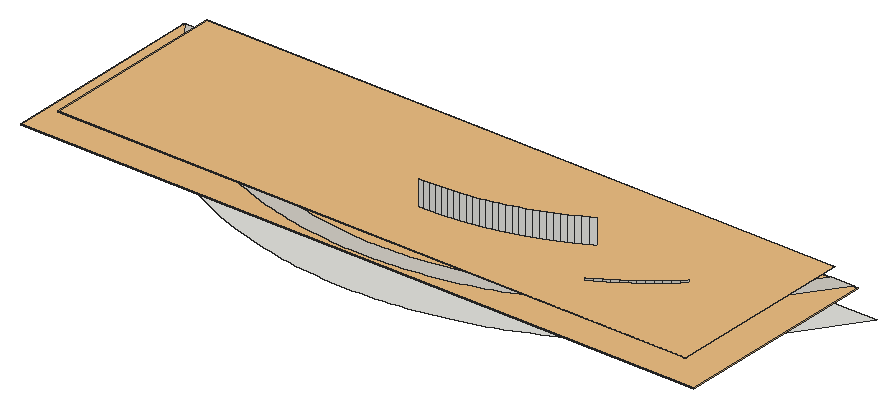
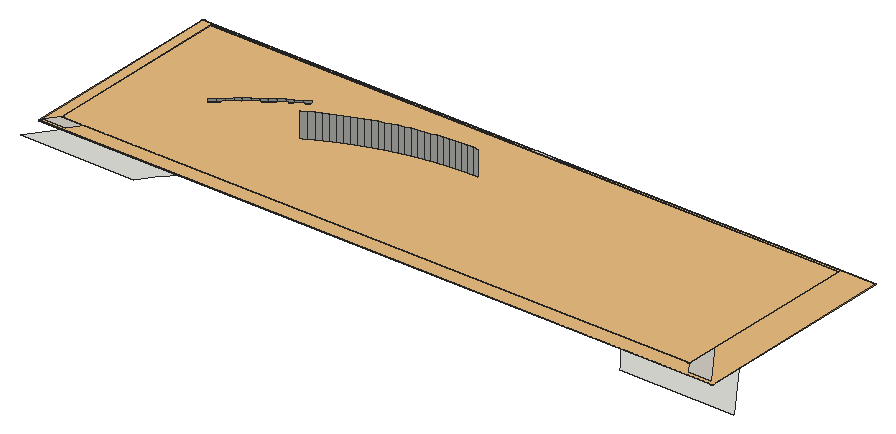
# SketchUp Ruby script. Lengths in inches.
U = 1.inch
M = Sketchup.active_model
def pt(a) = Geom::Point3d.new(a.map { |v| v * U })
def face(e, loops, mat)
  f = e.add_face(loops[0].map { |a| pt(a) })
  loops[1..].each { |l| e.add_face(l.map { |a| pt(a) }).erase! }
  f.material = f.back_material = mat if mat
  f
end
# faces: each face lists its corners as indices into pts; further lists are holes
def faces(e, pts, list, mat = nil) = list.each { |f| face(e, (f[0].is_a?(Array) ? f : [f]).map { |l| l.map { |i| pts[i] } }, mat) }
# xy, xz, yz: faces in a plane at the given z, y or x. An outline is a flat list of corners, or four numbers for a rectangle; further outlines are holes
def ring(l) = l.size == 4 ? [[l[0], l[1]], [l[2], l[1]], [l[2], l[3]], [l[0], l[3]]] : l.each_slice(2).to_a
def flat(e, list, mat, &to3) = list.each { |f| face(e, (f[0].is_a?(Array) ? f : [f]).map { |l| ring(l).map { |u, v| to3.(u, v) } }, mat) }
def xy(e, z, list, mat = nil) = flat(e, list, mat) { |x, y| [x, y, z] }
def xz(e, y, list, mat = nil) = flat(e, list, mat) { |x, z| [x, y, z] }
def yz(e, x, list, mat = nil) = flat(e, list, mat) { |y, z| [x, y, z] }
def lines(e, pts, list) = list.each { |a, b| e.add_line(pt(pts[a]), pt(pts[b])) }
# prism: a flat outline (further loops are holes) pulled along v
def prism(e, loops, v, mat = nil)
  f = face(e, loops, mat); d = Geom::Vector3d.new(v.map { |x| x * U })
  f.pushpull(f.normal.samedirection?(d) ? d.length : -d.length)
end
def box(e, o, s, mat = nil) = prism(e, [[o, [o[0] + s[0], o[1], o[2]], [o[0] + s[0], o[1] + s[1], o[2]], [o[0], o[1] + s[1], o[2]]]], [0, 0, s[2]], mat)
def at(x, y, z, deg = 0) = Geom::Transformation.translation(pt([x, y, z])) * Geom::Transformation.rotation(ORIGIN, Z_AXIS, deg.degrees)
def axes(o, x, y, z) = Geom::Transformation.new([*x, 0, *y, 0, *z, 0, *pt(o).to_a, 1])
def part(name) = M.definitions.add(name)
# library, detail: a bought-in or finely detailed component or shape, given as its bounding box
def library(name, o, s) = part(name).tap { |d| box(d.entities, o, s) }
def detail(e, o, s) = box(e.add_group.entities, o, s)
def put(e, d, t, mat = nil) = e.add_instance(d, t).tap { |i| i.material = mat if mat }
def group(e, t, mat = nil) = e.add_group.tap { |g| g.transformation = t; g.material = mat if mat }.entities
root = M.entities
M.materials.add("Arta-Ceramic-Moonstone-White-24x24-4K").color = [209, 205, 196]
c1 = library("Mesh Light\#8",[-0.5,-0.5,-0.1],[1,1,0.2])
c2 = library("Mesh Light\#7",[-0.5,-0.5,-0.1],[1,1,0.2])
xy(root,0,[[1024.28,79.26,1020.34,79.3,1016.39,79.42,1012.45,79.6,1008.51,79.87,1004.58,80.21,1000.66,80.625,996.74,81.12,992.84,81.68,988.94,82.32,985.0625,83.04,981.2,83.83,977.35,84.69,973.51,85.63,969.7,86.64,965.91,87.72,962.13,88.88,958.38,90.11,954.66,91.41,950.96,92.78,947.29,94.22,943.64,95.73,940.03,97.32,936.44,98.97,932.89,100.6875,929.37,102.47,925.89,104.33,922.44,106.25,919.03,108.24,915.66,110.29,912.33,112.4,909.04,114.58,905.8,116.82,902.59,119.13,899.44,121.49,896.32,123.92,893.26,126.4,890.24,128.95,887.27,131.55,884.36,134.2,881.49,136.92,878.68,139.68,875.92,142.5,873.21,145.375,870.5625,148.3,867.97,151.27,865.43,154.3,862.96,157.37,860.54,160.49,858.18,163.65,835.84,194.875,895.84,194.875,897.59,192.43,899.39,190.01,901.24,187.64,903.125,185.29,905.06,182.99,907.04,180.72,909.06,178.49,911.12,176.3,913.23,174.15,915.37,172.04,917.56,169.97,919.78,167.94,922.05,165.96,924.35,164.02,926.69,162.12,929.06,160.27,931.47,158.47,933.91,156.71,936.39,155,938.9,153.34,941.4375,151.72,944.01,150.16,946.61,148.64,949.24,147.18,951.89,145.76,954.58,144.4,957.28,143.09,960.02,141.83,962.78,140.625,965.56,139.47,968.36,138.37,971.18,137.32,974.02,136.33,976.88,135.4,979.76,134.51,982.65,133.6875,985.56,132.92,988.48,132.2,991.42,131.54,994.37,130.94,997.33,130.4,1000.3,129.91,1003.28,129.48,1006.26,129.1,1009.26,128.78,1012.25,128.52,1015.26,128.32,1018.26,128.18,1021.27,128.09,1024.28,128.0625,1027.29,128.09,1030.3,128.18,1033.3,128.32,1036.31,128.52,1039.31,128.78,1042.3,129.1,1045.28,129.48,1048.26,129.91,1051.23,130.4,1054.19,130.94,1057.14,131.54,1060.08,132.2,1063,132.92,1065.91,133.6875,1068.8,134.51,1071.68,135.4,1074.54,136.33,1077.38,137.32,1080.21,138.37,1083.01,139.47,1085.79,140.625,1088.54,141.83,1091.28,143.09,1093.99,144.4,1096.67,145.76,1099.33,147.18,1101.95,148.64,1104.55,150.16,1107.125,151.72,1109.67,153.34,1112.17,155,1114.65,156.71,1117.09,158.47,1119.5,160.27,1121.875,162.12,1124.21,164.02,1126.52,165.96,1128.78,167.94,1131,169.97,1133.19,172.04,1135.34,174.15,1137.44,176.3,1139.5,178.49,1141.52,180.72,1143.5,182.99,1145.4375,185.29,1147.33,187.64,1149.17,190.01,1150.97,192.43,1152.72,194.875,1212.72,194.875,1190.38,163.65,1188.02,160.49,1185.6,157.37,1183.13,154.3,1180.59,151.27,1178,148.3,1175.35,145.375,1172.65,142.5,1169.89,139.68,1167.07,136.92,1164.21,134.2,1161.29,131.55,1158.32,128.95,1155.3,126.4,1152.24,123.92,1149.125,121.49,1145.97,119.13,1142.76,116.82,1139.52,114.58,1136.23,112.4,1132.9,110.29,1129.53,108.24,1126.12,106.25,1122.67,104.33,1119.1875,102.47,1115.67,100.6875,1112.12,98.97,1108.54,97.32,1104.92,95.73,1101.28,94.22,1097.6,92.78,1093.9,91.41,1090.18,90.11,1086.43,88.88,1082.66,87.72,1078.86,86.64,1075.05,85.63,1071.21,84.69,1067.36,83.83,1063.5,83.04,1059.62,82.32,1055.72,81.68,1051.82,81.12,1047.9,80.625,1043.98,80.21,1040.05,79.87,1036.11,79.6,1032.17,79.42,1028.23,79.3]])
xy(root,12,[[1024.28,89.02,1028.04,89.06,1031.8,89.17,1035.55,89.35,1039.3,89.6,1043.05,89.92,1046.78,90.32,1050.51,90.79,1054.23,91.33,1057.94,91.9375,1061.64,92.62,1065.32,93.37,1068.99,94.19,1072.64,95.09,1076.27,96.05,1079.89,97.08,1083.48,98.18,1087.05,99.35,1090.6,100.59,1094.125,101.9,1097.62,103.27,1101.09,104.71,1104.54,106.22,1107.95,107.79,1111.33,109.43,1114.68,111.13,1118,112.9,1121.29,114.73,1124.53,116.62,1127.74,118.57,1130.92,120.59,1134.05,122.67,1137.14,124.8,1140.19,127,1143.2,129.25,1146.17,131.56,1149.09,133.93,1151.96,136.35,1154.79,138.83,1157.57,141.36,1160.3,143.94,1162.98,146.58,1165.6,149.26,1168.18,152,1170.7,154.78,1173.17,157.62,1175.59,160.5,1177.95,163.42,1180.25,166.39,1182.5,169.41,1200.72,194.875,1188.72,194.875,1174.61,175.16,1172.48,172.3,1170.29,169.48,1168.05,166.7,1165.76,163.96,1163.41,161.27,1161.01,158.62,1158.5625,156.02,1156.07,153.47,1153.52,150.96,1150.93,148.51,1148.29,146.1,1145.6,143.75,1142.87,141.45,1140.09,139.2,1137.28,137.01,1134.42,134.86,1131.52,132.78,1128.58,130.75,1125.6,128.78,1122.59,126.86,1119.54,125,1116.45,123.21,1113.33,121.47,1110.18,119.79,1107,118.17,1103.78,116.62,1100.54,115.12,1097.27,113.69,1093.97,112.32,1090.64,111.02,1087.3,109.77,1083.92,108.6,1080.53,107.49,1077.12,106.4375,1073.68,105.46,1070.23,104.54,1066.76,103.7,1063.28,102.91,1059.78,102.2,1056.26,101.55,1052.74,100.97,1049.21,100.46,1045.66,100.02,1042.11,99.64,1038.55,99.33,1034.99,99.09,1031.42,98.92,1027.85,98.82,1024.28,98.78,1020.71,98.82,1017.14,98.92,1013.57,99.09,1010.01,99.33,1006.45,99.64,1002.9,100.02,999.36,100.46,995.82,100.97,992.3,101.55,988.79,102.2,985.29,102.91,981.8,103.7,978.33,104.54,974.88,105.46,971.45,106.4375,968.03,107.49,964.64,108.6,961.27,109.77,957.92,111.02,954.59,112.32,951.29,113.69,948.02,115.12,944.78,116.62,941.56,118.17,938.38,119.79,935.23,121.47,932.11,123.21,929.02,125,925.97,126.86,922.96,128.78,919.98,130.75,917.04,132.78,914.14,134.86,911.28,137.01,908.47,139.2,905.69,141.45,902.96,143.75,900.28,146.1,897.64,148.51,895.04,150.96,892.5,153.47,890,156.02,887.55,158.62,885.15,161.27,882.81,163.96,880.51,166.7,878.27,169.48,876.08,172.3,873.95,175.16,859.84,194.875,847.84,194.875,866.06,169.41,868.31,166.39,870.61,163.42,872.97,160.5,875.39,157.62,877.86,154.78,880.38,152,882.96,149.26,885.59,146.58,888.27,143.94,891,141.36,893.77,138.83,896.6,136.35,899.48,133.93,902.4,131.56,905.36,129.25,908.37,127,911.42,124.8,914.51,122.67,917.65,120.59,920.82,118.57,924.03,116.62,927.28,114.73,930.56,112.9,933.875,111.13,937.23,109.43,940.61,107.79,944.02,106.22,947.47,104.71,950.9375,103.27,954.4375,101.9,957.96,100.59,961.51,99.35,965.08,98.18,968.68,97.08,972.29,96.05,975.92,95.09,979.57,94.19,983.24,93.37,986.92,92.62,990.62,91.9375,994.33,91.33,998.05,90.79,1001.78,90.32,1005.52,89.92,1009.26,89.6,1013.01,89.35,1016.77,89.17,1020.52,89.06]],"Arta-Ceramic-Moonstone-White-24x24-4K")
p = [[1152.24,123.92,5],[1152.24,123.92,0],[1155.3,126.4,0],[1155.3,126.4,5],[1158.32,128.95,0],[1158.32,128.95,5],
  [1024.28,128.0625,0],[1024.28,128.0625,30],[1027.29,128.09,30],[1027.29,128.09,0],[1030.3,128.18,30],[1030.3,128.18,0],
  [1033.3,128.32,30],[1033.3,128.32,0],[1036.31,128.52,30],[1036.31,128.52,0],[1039.31,128.78,30],[1039.31,128.78,0],
  [1042.3,129.1,30],[1042.3,129.1,0],[1161.29,131.55,0],[1161.29,131.55,5],[1045.28,129.48,30],[1045.28,129.48,0],
  [1048.26,129.91,30],[1048.26,129.91,0],[1051.23,130.4,30],[1051.23,130.4,0],[1054.19,130.94,30],[1054.19,130.94,0],
  [1057.14,131.54,30],[1057.14,131.54,0],[1060.08,132.2,30],[1060.08,132.2,0],[1164.21,134.2,0],[1164.21,134.2,5],
  [1063,132.92,30],[1063,132.92,0],[1065.91,133.6875,30],[1065.91,133.6875,0],[1068.8,134.51,30],[1068.8,134.51,0],
  [1167.07,136.92,0],[1167.07,136.92,5],[1071.68,135.4,30],[1071.68,135.4,0],[1074.54,136.33,30],[1074.54,136.33,0],
  [1077.38,137.32,30],[1077.38,137.32,0],[1169.89,139.68,0],[1169.89,139.68,5],[1080.21,138.37,30],[1080.21,138.37,0],
  [1083.01,139.47,30],[1083.01,139.47,0],[1085.79,140.625,30],[1085.79,140.625,0],[1172.65,142.5,0],[1172.65,142.5,5],
  [1088.54,141.83,30],[1088.54,141.83,0],[1091.28,143.09,30],[1091.28,143.09,0],[1175.35,145.375,0],[1175.35,145.375,5],
  [1093.99,144.4,30],[1093.99,144.4,0],[1096.67,145.76,30],[1096.67,145.76,0],[1178,148.3,0],[1178,148.3,5],
  [1099.33,147.18,30],[1099.33,147.18,0],[1101.95,148.64,30],[1101.95,148.64,0],[1152.74,123.28,6],[1152.74,123.28,5],
  [1155.82,125.78,5],[1155.82,125.78,6],[1158.85,128.33,5],[1158.85,128.33,6],[1161.83,130.94,5],[1161.83,130.94,6],
  [1164.76,133.61,5],[1164.76,133.61,6],[1167.64,136.33,5],[1167.64,136.33,6],[1170.46,139.11,5],[1170.46,139.11,6],
  [1173.23,141.94,5],[1173.23,141.94,6],[1175.95,144.82,5],[1175.95,144.82,6],[1178.61,147.76,5],[1178.61,147.76,6],
  [1134.05,122.67,11],[1134.05,122.67,6],[1137.14,124.8,6],[1137.14,124.8,11],[1140.19,127,6],[1140.19,127,11],
  [1143.2,129.25,6],[1143.2,129.25,11],[1146.17,131.56,6],[1146.17,131.56,11],[1149.09,133.93,6],[1149.09,133.93,11],
  [1151.96,136.35,6],[1151.96,136.35,11],[1154.79,138.83,6],[1154.79,138.83,11],[1157.57,141.36,6],[1157.57,141.36,11],
  [1160.3,143.94,6],[1160.3,143.94,11],[1162.98,146.58,6],[1162.98,146.58,11],[1165.6,149.26,6],[1165.6,149.26,11],
  [1134.5,121.99,12],[1134.5,121.99,11],[1137.61,124.14,11],[1137.61,124.14,12],[1140.67,126.34,11],[1140.67,126.34,12],
  [1143.7,128.6,11],[1143.7,128.6,12],[1146.67,130.92,11],[1146.67,130.92,12],[1149.6,133.3,11],[1149.6,133.3,12],
  [1152.49,135.73,11],[1152.49,135.73,12],[1155.33,138.22,11],[1155.33,138.22,12],[1158.12,140.76,11],[1158.12,140.76,12],
  [1160.86,143.35,11],[1160.86,143.35,12],[1163.55,146,11],[1163.55,146,12],[1166.19,148.7,11],[1166.19,148.7,12],
  [1116.45,123.21,17],[1116.45,123.21,12],[1119.54,125,12],[1119.54,125,17],[1122.59,126.86,12],[1122.59,126.86,17],
  [1125.6,128.78,12],[1125.6,128.78,17],[1128.58,130.75,12],[1128.58,130.75,17],[1131.52,132.78,12],[1131.52,132.78,17],
  [1134.42,134.86,12],[1134.42,134.86,17],[1137.28,137.01,12],[1137.28,137.01,17],[1140.09,139.2,12],[1140.09,139.2,17],
  [1142.87,141.45,12],[1142.87,141.45,17],[1145.6,143.75,12],[1145.6,143.75,17],[1148.29,146.1,12],[1148.29,146.1,17],
  [1150.93,148.51,12],[1150.93,148.51,17],[1116.86,122.5,18],[1116.86,122.5,17],[1119.95,124.31,17],[1119.95,124.31,18],
  [1123.02,126.17,17],[1123.02,126.17,18],[1126.05,128.09,17],[1126.05,128.09,18],[1129.04,130.08,17],[1129.04,130.08,18],
  [1131.99,132.11,17],[1131.99,132.11,18],[1134.9,134.21,17],[1134.9,134.21,18],[1137.77,136.36,17],[1137.77,136.36,18],
  [1140.6,138.5625,17],[1140.6,138.5625,18],[1143.39,140.82,17],[1143.39,140.82,18],[1146.13,143.13,17],[1146.13,143.13,18],
  [1148.83,145.5,17],[1148.83,145.5,18],[1151.48,147.91,17],[1151.48,147.91,18]]
faces(root,p,[[0,1,2,3],[3,2,4,5],[5,4,20,21],[21,20,34,35],[35,34,42,43],[43,42,50,51],[51,50,58,59],[59,58,64,65],
  [65,64,70,71],[76,77,78,79],[79,78,80,81],[81,80,82,83],[83,82,84,85],[85,84,86,87],[87,86,88,89],[89,88,90,91],
  [91,90,92,93],[93,92,94,95],[96,97,98,99],[99,98,100,101],[101,100,102,103],[103,102,104,105],[105,104,106,107],[107,106,108,109],
  [109,108,110,111],[111,110,112,113],[113,112,114,115],[115,114,116,117],[117,116,118,119],[120,121,122,123],[123,122,124,125],[125,124,126,127],
  [127,126,128,129],[129,128,130,131],[131,130,132,133],[133,132,134,135],[135,134,136,137],[137,136,138,139],[139,138,140,141],[141,140,142,143],
  [144,145,146,147],[147,146,148,149],[149,148,150,151],[151,150,152,153],[153,152,154,155],[155,154,156,157],[157,156,158,159],[159,158,160,161],
  [161,160,162,163],[163,162,164,165],[165,164,166,167],[167,166,168,169],[170,171,172,173],[173,172,174,175],[175,174,176,177],[177,176,178,179],
  [179,178,180,181],[181,180,182,183],[183,182,184,185],[185,184,186,187],[187,186,188,189],[189,188,190,191],[191,190,192,193],[193,192,194,195]],"Arta-Ceramic-Moonstone-White-24x24-4K")
faces(root,p,[[6,7,8,9],[9,8,10,11],[11,10,12,13],[13,12,14,15],[15,14,16,17],[17,16,18,19],[19,18,22,23],[23,22,24,25],
  [25,24,26,27],[27,26,28,29],[29,28,30,31],[31,30,32,33],[33,32,36,37],[37,36,38,39],[39,38,40,41],[41,40,44,45],
  [45,44,46,47],[47,46,48,49],[49,48,52,53],[53,52,54,55],[55,54,56,57],[57,56,60,61],[61,60,62,63],[63,62,66,67],
  [67,66,68,69],[69,68,72,73],[73,72,74,75]])
g1 = group(root,at(846.84,88.21,11))
xy(g1,0,[[177.4375,0,173.66,0.04,169.89,0.14,166.12,0.33,162.36,0.58,158.6,0.9,154.84,1.3,151.1,1.77,147.36,2.3125,143.64,2.93,139.93,3.61,136.23,4.36,132.55,5.19,128.88,6.09,125.23,7.05,121.6,8.09,117.99,9.2,114.41,10.37,110.84,11.62,107.3,12.93,103.79,14.31,100.31,15.75,96.85,17.27,93.42,18.85,90.02,20.49,86.66,22.2,83.33,23.97,80.03,25.8125,76.77,27.71,73.55,29.67,70.36,31.7,67.21,33.78,64.11,35.93,61.04,38.13,58.02,40.39,55.05,42.71,52.11,45.09,49.23,47.52,46.39,50.01,43.6,52.55,40.86,55.14,38.17,57.79,35.53,60.49,32.94,63.24,30.41,66.03,27.93,68.88,25.5,71.77,23.13,74.71,20.82,77.69,18.56,80.72,0,106.66,1,106.66,19.22,81.2,21.47,78.18,23.77,75.21,26.13,72.29,28.54,69.41,31.01,66.57,33.54,63.79,36.11,61.05,38.74,58.37,41.42,55.73,44.15,53.15,46.93,50.62,49.76,48.14,52.63,45.72,55.55,43.35,58.52,41.04,61.53,38.79,64.58,36.59,67.67,34.46,70.8,32.38,73.97,30.36,77.19,28.41,80.43,26.52,83.72,24.6875,87.03,22.92,90.38,21.22,93.77,19.58,97.18,18.01,100.625,16.5,104.1,15.0625,107.59,13.6875,111.12,12.38,114.67,11.14,118.24,9.97,121.83,8.87,125.45,7.84,129.08,6.875,132.73,5.98,136.4,5.16,140.08,4.41,143.78,3.73,147.49,3.12,151.21,2.58,154.94,2.11,158.67,1.71,162.42,1.39,166.17,1.14,169.92,0.96,173.68,0.85,177.4375,0.8125,181.2,0.85,184.95,0.96,188.71,1.14,192.46,1.39,196.2,1.71,199.94,2.11,203.67,2.58,207.39,3.12,211.1,3.73,214.79,4.41,218.48,5.16,222.14,5.98,225.79,6.875,229.43,7.84,233.04,8.87,236.64,9.97,240.21,11.14,243.76,12.38,247.28,13.6875,250.78,15.0625,254.25,16.5,257.69,18.01,261.11,19.58,264.49,21.22,267.84,22.92,271.16,24.6875,274.44,26.52,277.69,28.41,280.9,30.36,284.07,32.38,287.21,34.46,290.3,36.59,293.35,38.79,296.36,41.04,299.32,43.35,302.24,45.72,305.12,48.14,307.94,50.62,310.72,53.15,313.45,55.73,316.13,58.37,318.76,61.05,321.34,63.79,323.86,66.57,326.33,69.41,328.75,72.29,331.11,75.21,333.41,78.18,335.65,81.2,353.875,106.66,354.2,107.12,354.86,106.65,336.31,80.72,334.06,77.69,331.74,74.71,329.375,71.77,326.95,68.88,324.47,66.03,321.94,63.24,319.35,60.49,316.71,57.79,314.02,55.14,311.28,52.55,308.49,50.01,305.65,47.52,302.76,45.09,299.83,42.71,296.85,40.39,293.83,38.13,290.77,35.93,287.66,33.78,284.52,31.7,281.33,29.67,278.11,27.71,274.84,25.8125,271.55,23.97,268.22,22.2,264.85,20.49,261.46,18.85,258.03,17.27,254.57,15.75,251.08,14.31,247.57,12.93,244.03,11.62,240.47,10.37,236.88,9.2,233.27,8.09,229.64,7.05,226,6.09,222.33,5.19,218.65,4.36,214.95,3.61,211.24,2.93,207.51,2.3125,203.78,1.77,200.03,1.3,196.28,0.9,192.52,0.58,188.75,0.33,184.98,0.14,181.21,0.04]],"Arta-Ceramic-Moonstone-White-24x24-4K")
put(g1,c1,axes([177.43,53.5625,0],[355.86372,0,0],[0,108.12208,0],[0,0,1]))
g2 = group(root,at(858.84,97.97,17))
xy(g2,0,[[165.4375,0,161.85,0.03,158.27,0.14,154.68,0.31,151.1,0.55,147.53,0.86,143.96,1.24,140.4,1.68,136.85,2.2,133.31,2.78,129.79,3.43,126.27,4.15,122.77,4.93,119.29,5.79,115.82,6.7,112.37,7.6875,108.94,8.74,105.53,9.86,102.15,11.04,98.78,12.29,95.45,13.6,92.13,14.97,88.85,16.41,85.59,17.91,82.36,19.47,79.16,21.1,76,22.78,72.86,24.53,69.76,26.34,66.7,28.2,63.67,30.125,60.68,32.11,57.73,34.14,54.82,36.24,51.95,38.39,49.12,40.59,46.33,42.85,43.59,45.16,40.89,47.53,38.24,49.94,35.63,52.41,33.08,54.92,30.57,57.49,28.11,60.1,25.7,62.76,23.34,65.46,21.04,68.21,18.79,71,16.59,73.84,14.45,76.71,0,96.9,1,96.9,15.1,77.19,17.24,74.33,19.43,71.51,21.67,68.73,23.96,65.99,26.31,63.3,28.71,60.65,31.15,58.05,33.65,55.5,36.2,52.99,38.79,50.54,41.43,48.13,44.12,45.78,46.85,43.48,49.625,41.23,52.44,39.04,55.3,36.89,58.2,34.81,61.14,32.78,64.12,30.81,67.13,28.89,70.18,27.03,73.27,25.24,76.39,23.5,79.54,21.82,82.72,20.2,85.9375,18.65,89.18,17.15,92.45,15.72,95.75,14.35,99.07,13.05,102.42,11.8,105.79,10.63,109.1875,9.52,112.6,8.47,116.04,7.49,119.49,6.57,122.96,5.73,126.44,4.94,129.94,4.23,133.45,3.58,136.98,3,140.51,2.49,144.06,2.05,147.61,1.67,151.17,1.36,154.73,1.12,158.3,0.95,161.87,0.85,165.4375,0.8125,169.01,0.85,172.58,0.95,176.15,1.12,179.71,1.36,183.27,1.67,186.82,2.05,190.36,2.49,193.9,3,197.42,3.58,200.93,4.23,204.43,4.94,207.92,5.73,211.39,6.57,214.84,7.49,218.27,8.47,221.6875,9.52,225.08,10.63,228.45,11.8,231.8,13.05,235.125,14.35,238.42,15.72,241.7,17.15,244.9375,18.65,248.15,20.2,251.34,21.82,254.49,23.5,257.61,25.24,260.7,27.03,263.75,28.89,266.76,30.81,269.74,32.78,272.68,34.81,275.57,36.89,278.43,39.04,281.25,41.23,284.02,43.48,286.76,45.78,289.44,48.13,292.08,50.54,294.68,52.99,297.22,55.5,299.72,58.05,302.17,60.65,304.57,63.3,306.91,65.99,309.21,68.73,311.45,71.51,313.64,74.33,315.77,77.19,329.875,96.9,330.24,97.41,330.9,96.94,316.43,76.71,314.29,73.84,312.09,71,309.84,68.21,307.53,65.46,305.17,62.76,302.77,60.1,300.31,57.49,297.8,54.92,295.24,52.41,292.64,49.94,289.98,47.53,287.29,45.16,284.54,42.85,281.76,40.59,278.93,38.39,276.06,36.24,273.14,34.14,270.19,32.11,267.2,30.125,264.18,28.2,261.11,26.34,258.01,24.53,254.88,22.78,251.71,21.1,248.51,19.47,245.29,17.91,242.03,16.41,238.74,14.97,235.43,13.6,232.09,12.29,228.73,11.04,225.34,9.86,221.93,8.74,218.5,7.6875,215.05,6.7,211.59,5.79,208.1,4.93,204.6,4.15,201.09,3.43,197.56,2.78,194.02,2.2,190.47,1.68,186.91,1.24,183.34,0.86,179.77,0.55,176.19,0.31,172.61,0.14,169.02,0.03]],"Arta-Ceramic-Moonstone-White-24x24-4K")
put(g2,c2,axes([165.45,48.71,0],[331.90009,0,0],[0,98.4132,0],[0,0,1]))
